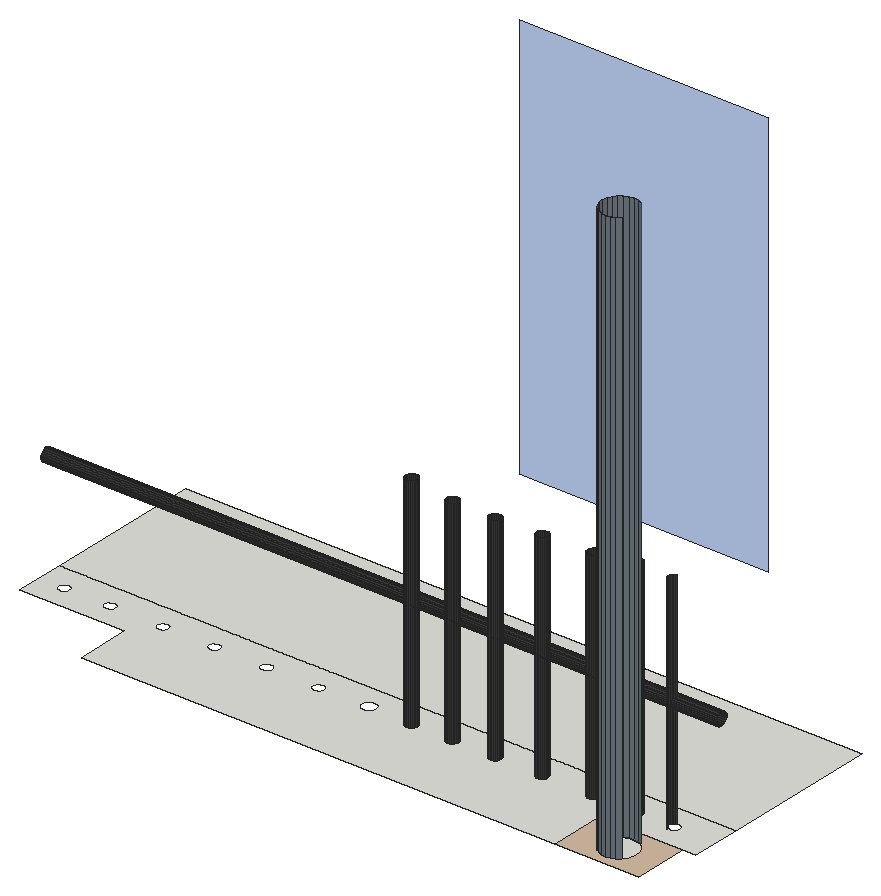
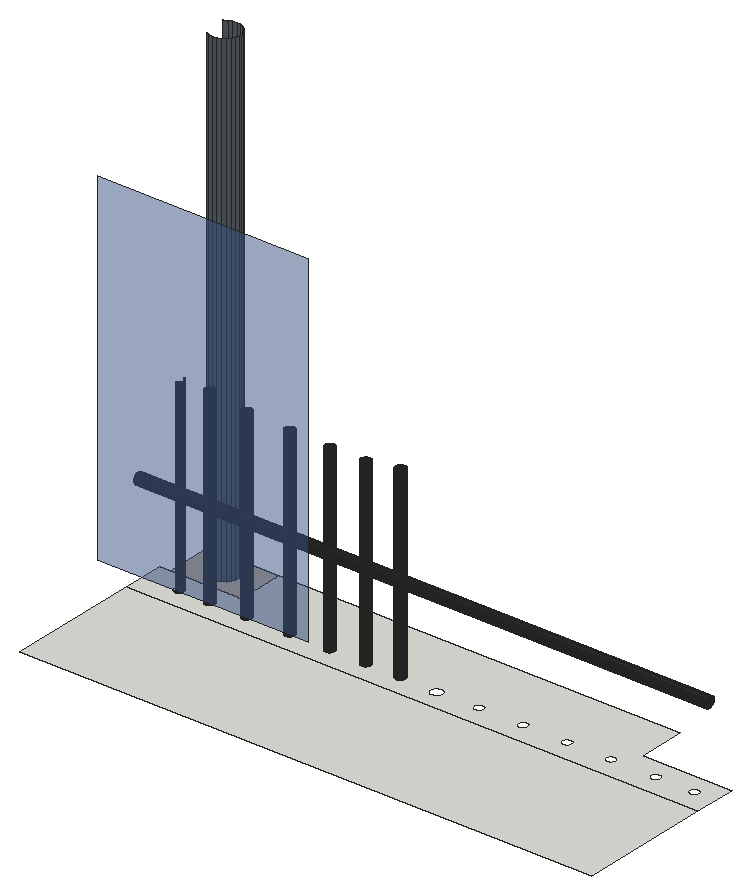
# SketchUp Ruby script. Lengths in inches.
U = 1.inch
M = Sketchup.active_model
def pt(a) = Geom::Point3d.new(a.map { |v| v * U })
def face(e, loops, mat)
  f = e.add_face(loops[0].map { |a| pt(a) })
  loops[1..].each { |l| e.add_face(l.map { |a| pt(a) }).erase! }
  f.material = f.back_material = mat if mat
  f
end
# faces: each face lists its corners as indices into pts; further lists are holes
def faces(e, pts, list, mat = nil) = list.each { |f| face(e, (f[0].is_a?(Array) ? f : [f]).map { |l| l.map { |i| pts[i] } }, mat) }
# xy, xz, yz: faces in a plane at the given z, y or x. An outline is a flat list of corners, or four numbers for a rectangle; further outlines are holes
def ring(l) = l.size == 4 ? [[l[0], l[1]], [l[2], l[1]], [l[2], l[3]], [l[0], l[3]]] : l.each_slice(2).to_a
def flat(e, list, mat, &to3) = list.each { |f| face(e, (f[0].is_a?(Array) ? f : [f]).map { |l| ring(l).map { |u, v| to3.(u, v) } }, mat) }
def xy(e, z, list, mat = nil) = flat(e, list, mat) { |x, y| [x, y, z] }
def xz(e, y, list, mat = nil) = flat(e, list, mat) { |x, z| [x, y, z] }
def yz(e, x, list, mat = nil) = flat(e, list, mat) { |y, z| [x, y, z] }
def lines(e, pts, list) = list.each { |a, b| e.add_line(pt(pts[a]), pt(pts[b])) }
# prism: a flat outline (further loops are holes) pulled along v
def prism(e, loops, v, mat = nil)
  f = face(e, loops, mat); d = Geom::Vector3d.new(v.map { |x| x * U })
  f.pushpull(f.normal.samedirection?(d) ? d.length : -d.length)
end
def box(e, o, s, mat = nil) = prism(e, [[o, [o[0] + s[0], o[1], o[2]], [o[0] + s[0], o[1] + s[1], o[2]], [o[0], o[1] + s[1], o[2]]]], [0, 0, s[2]], mat)
def at(x, y, z, deg = 0) = Geom::Transformation.translation(pt([x, y, z])) * Geom::Transformation.rotation(ORIGIN, Z_AXIS, deg.degrees)
def axes(o, x, y, z) = Geom::Transformation.new([*x, 0, *y, 0, *z, 0, *pt(o).to_a, 1])
def part(name) = M.definitions.add(name)
# library, detail: a bought-in or finely detailed component or shape, given as its bounding box
def library(name, o, s) = part(name).tap { |d| box(d.entities, o, s) }
def detail(e, o, s) = box(e.add_group.entities, o, s)
def put(e, d, t, mat = nil) = e.add_instance(d, t).tap { |i| i.material = mat if mat }
def group(e, t, mat = nil) = e.add_group.tap { |g| g.transformation = t; g.material = mat if mat }.entities
root = M.entities
M.materials.add("[Color M07]").color = [58, 58, 58]
M.materials.add("[Formica Laminate Light]").color = [213, 189, 164]
M.materials.add("[Formica Speckled Grey]").color = [112, 125, 132]
M.materials.add("[Translucent Glass Blue]").color = [85, 126, 201]
M.materials["[Translucent Glass Blue]"].alpha = 0.5
xy(root,273.71,[[[59.49,83.35,115.23,83.35,115.23,89.73,126.66,89.73,126.66,95.59,47.16,95.59,47.16,89.73,59.49,89.73],[85.8,91.86,85.57,91.89,85.36,91.97,85.18,92.11,85.04,92.29,84.95,92.5,84.92,92.73,84.95,92.96,85.04,93.17,85.18,93.35,85.36,93.49,85.57,93.58,85.8,93.61,86.02,93.58,86.24,93.49,86.42,93.35,86.56,93.17,86.64,92.96,86.67,92.73,86.64,92.5,86.56,92.29,86.42,92.11,86.24,91.97,86.02,91.89],[50.09,91.87,49.91,91.89,49.75,91.96,49.61,92.07,49.5,92.21,49.43,92.38,49.4,92.56,49.43,92.73,49.5,92.9,49.61,93.04,49.75,93.15,49.91,93.22,50.09,93.24,50.27,93.22,50.4375,93.15,50.58,93.04,50.6875,92.9,50.76,92.73,50.78,92.56,50.76,92.38,50.6875,92.21,50.58,92.07,50.4375,91.96,50.27,91.89],[55.47,91.87,55.29,91.89,55.125,91.96,54.98,92.07,54.87,92.21,54.8,92.38,54.78,92.56,54.8,92.73,54.87,92.9,54.98,93.04,55.125,93.15,55.29,93.22,55.47,93.24,55.64,93.22,55.8125,93.15,55.95,93.04,56.0625,92.9,56.13,92.73,56.15,92.56,56.13,92.38,56.0625,92.21,55.95,92.07,55.8125,91.96,55.64,91.89],[67.78,91.87,67.6,91.89,67.4375,91.96,67.29,92.07,67.18,92.21,67.12,92.38,67.09,92.56,67.12,92.73,67.18,92.9,67.29,93.04,67.4375,93.15,67.6,93.22,67.78,93.24,67.96,93.22,68.125,93.15,68.27,93.04,68.375,92.9,68.44,92.73,68.47,92.56,68.44,92.38,68.375,92.21,68.27,92.07,68.125,91.96,67.96,91.89],[61.72,91.87,61.54,91.89,61.375,91.96,61.23,92.07,61.12,92.21,61.05,92.38,61.03,92.56,61.05,92.73,61.12,92.9,61.23,93.04,61.375,93.15,61.54,93.22,61.72,93.24,61.89,93.22,62.0625,93.15,62.2,93.04,62.3125,92.9,62.38,92.73,62.4,92.56,62.38,92.38,62.3125,92.21,62.2,92.07,62.0625,91.96,61.89,91.89],[73.9,91.87,73.73,91.89,73.5625,91.96,73.42,92.07,73.31,92.21,73.24,92.38,73.22,92.56,73.24,92.73,73.31,92.9,73.42,93.04,73.5625,93.15,73.73,93.22,73.9,93.24,74.08,93.22,74.25,93.15,74.39,93.04,74.5,92.9,74.57,92.73,74.59,92.56,74.57,92.38,74.5,92.21,74.39,92.07,74.25,91.96,74.08,91.89],[121.84,91.87,121.66,91.89,121.5,91.96,121.36,92.07,121.25,92.21,121.18,92.38,121.15,92.56,121.18,92.73,121.25,92.9,121.36,93.04,121.5,93.15,121.66,93.22,121.84,93.24,122.02,93.22,122.1875,93.15,122.33,93.04,122.4375,92.9,122.51,92.73,122.53,92.56,122.51,92.38,122.4375,92.21,122.33,92.07,122.1875,91.96,122.02,91.89],[90.97,91.87,90.79,91.89,90.625,91.96,90.48,92.07,90.37,92.21,90.3,92.38,90.28,92.56,90.3,92.73,90.37,92.9,90.48,93.04,90.625,93.15,90.79,93.22,90.97,93.24,91.14,93.22,91.3125,93.15,91.45,93.04,91.5625,92.9,91.63,92.73,91.65,92.56,91.63,92.38,91.5625,92.21,91.45,92.07,91.3125,91.96,91.14,91.89],[117.47,91.87,117.29,91.89,117.125,91.96,116.98,92.07,116.87,92.21,116.8,92.38,116.78,92.56,116.8,92.73,116.87,92.9,116.98,93.04,117.125,93.15,117.29,93.22,117.47,93.24,117.64,93.22,117.8125,93.15,117.95,93.04,118.0625,92.9,118.13,92.73,118.15,92.56,118.13,92.38,118.0625,92.21,117.95,92.07,117.8125,91.96,117.64,91.89],[95.78,91.87,95.6,91.89,95.4375,91.96,95.29,92.07,95.18,92.21,95.12,92.38,95.09,92.56,95.12,92.73,95.18,92.9,95.29,93.04,95.4375,93.15,95.6,93.22,95.78,93.24,95.96,93.22,96.125,93.15,96.27,93.04,96.375,92.9,96.44,92.73,96.47,92.56,96.44,92.38,96.375,92.21,96.27,92.07,96.125,91.96,95.96,91.89],[112.34,91.87,112.16,91.89,112,91.96,111.86,92.07,111.75,92.21,111.68,92.38,111.65,92.56,111.68,92.73,111.75,92.9,111.86,93.04,112,93.15,112.16,93.22,112.34,93.24,112.52,93.22,112.6875,93.15,112.83,93.04,112.9375,92.9,113.01,92.73,113.03,92.56,113.01,92.38,112.9375,92.21,112.83,92.07,112.6875,91.96,112.52,91.89],[100.78,91.87,100.6,91.89,100.4375,91.96,100.29,92.07,100.18,92.21,100.12,92.38,100.09,92.56,100.12,92.73,100.18,92.9,100.29,93.04,100.4375,93.15,100.6,93.22,100.78,93.24,100.96,93.22,101.125,93.15,101.27,93.04,101.375,92.9,101.44,92.73,101.47,92.56,101.44,92.38,101.375,92.21,101.27,92.07,101.125,91.96,100.96,91.89],[106.34,91.87,106.16,91.89,106,91.96,105.86,92.07,105.75,92.21,105.68,92.38,105.65,92.56,105.68,92.73,105.75,92.9,105.86,93.04,106,93.15,106.16,93.22,106.34,93.24,106.52,93.22,106.6875,93.15,106.83,93.04,106.9375,92.9,107.01,92.73,107.03,92.56,107.01,92.38,106.9375,92.21,106.83,92.07,106.6875,91.96,106.52,91.89],[80.03,91.87,79.85,91.89,79.6875,91.96,79.54,92.07,79.43,92.21,79.37,92.38,79.34,92.56,79.37,92.73,79.43,92.9,79.54,93.04,79.6875,93.15,79.85,93.22,80.03,93.24,80.21,93.22,80.375,93.15,80.52,93.04,80.625,92.9,80.69,92.73,80.72,92.56,80.69,92.38,80.625,92.21,80.52,92.07,80.375,91.96,80.21,91.89]],[120.4,84.29,119.86,84.36,119.37,84.57,118.9375,84.89,118.61,85.32,118.41,85.82,118.33,86.35,118.41,86.89,118.61,87.38,118.9375,87.8125,119.37,88.14,119.86,88.35,120.4,88.42,120.93,88.35,121.43,88.14,121.86,87.8125,122.18,87.38,122.39,86.89,122.46,86.35,122.39,85.82,122.18,85.32,121.86,84.89,121.43,84.57,120.93,84.36],[90.97,91.87,90.79,91.89,90.625,91.96,90.48,92.07,90.37,92.21,90.3,92.38,90.28,92.56,90.3,92.73,90.37,92.9,90.48,93.04,90.625,93.15,90.79,93.22,90.97,93.24,91.14,93.22,91.3125,93.15,91.45,93.04,91.5625,92.9,91.63,92.73,91.65,92.56,91.63,92.38,91.5625,92.21,91.45,92.07,91.3125,91.96,91.14,91.89],[95.78,91.87,95.6,91.89,95.4375,91.96,95.29,92.07,95.18,92.21,95.12,92.38,95.09,92.56,95.12,92.73,95.18,92.9,95.29,93.04,95.4375,93.15,95.6,93.22,95.78,93.24,95.96,93.22,96.125,93.15,96.27,93.04,96.375,92.9,96.44,92.73,96.47,92.56,96.44,92.38,96.375,92.21,96.27,92.07,96.125,91.96,95.96,91.89],[100.78,91.87,100.6,91.89,100.4375,91.96,100.29,92.07,100.18,92.21,100.12,92.38,100.09,92.56,100.12,92.73,100.18,92.9,100.29,93.04,100.4375,93.15,100.6,93.22,100.78,93.24,100.96,93.22,101.125,93.15,101.27,93.04,101.375,92.9,101.44,92.73,101.47,92.56,101.44,92.38,101.375,92.21,101.27,92.07,101.125,91.96,100.96,91.89],
  [106.34,91.87,106.16,91.89,106,91.96,105.86,92.07,105.75,92.21,105.68,92.38,105.65,92.56,105.68,92.73,105.75,92.9,105.86,93.04,106,93.15,106.16,93.22,106.34,93.24,106.52,93.22,106.6875,93.15,106.83,93.04,106.9375,92.9,107.01,92.73,107.03,92.56,107.01,92.38,106.9375,92.21,106.83,92.07,106.6875,91.96,106.52,91.89],[112.34,91.87,112.16,91.89,112,91.96,111.86,92.07,111.75,92.21,111.68,92.38,111.65,92.56,111.68,92.73,111.75,92.9,111.86,93.04,112,93.15,112.16,93.22,112.34,93.24,112.52,93.22,112.6875,93.15,112.83,93.04,112.9375,92.9,113.01,92.73,113.03,92.56,113.01,92.38,112.9375,92.21,112.83,92.07,112.6875,91.96,112.52,91.89],[117.47,91.87,117.29,91.89,117.125,91.96,116.98,92.07,116.87,92.21,116.8,92.38,116.78,92.56,116.8,92.73,116.87,92.9,116.98,93.04,117.125,93.15,117.29,93.22,117.47,93.24,117.64,93.22,117.8125,93.15,117.95,93.04,118.0625,92.9,118.13,92.73,118.15,92.56,118.13,92.38,118.0625,92.21,117.95,92.07,117.8125,91.96,117.64,91.89],[47.16,95.59,126.66,114.1]])
xy(root,273.71,[[[115.23,83.35,125.11,89.73],[120.4,84.29,119.86,84.36,119.37,84.57,118.9375,84.89,118.61,85.32,118.41,85.82,118.33,86.35,118.41,86.89,118.61,87.38,118.9375,87.8125,119.37,88.14,119.86,88.35,120.4,88.42,120.93,88.35,121.43,88.14,121.86,87.8125,122.18,87.38,122.39,86.89,122.46,86.35,122.39,85.82,122.18,85.32,121.86,84.89,121.43,84.57,120.93,84.36]]],"[Formica Laminate Light]")
xz(root,114.1,[[86.49,288.95,115.77,336.88]],"[Translucent Glass Blue]")
p = [[119.86,84.36,273.71],[120.4,84.29,273.71],[120.4,84.29,341.31],[119.86,84.36,341.31],[120.93,84.36,273.71],[120.93,84.36,341.31],
  [119.37,84.57,273.71],[119.37,84.57,341.31],[121.43,84.57,273.71],[121.43,84.57,341.31],[118.9375,84.89,273.71],[118.9375,84.89,341.31],
  [121.86,84.89,273.71],[121.86,84.89,341.31],[118.61,85.32,273.71],[118.61,85.32,341.31],[118.41,85.82,273.71],[118.41,85.82,341.31],
  [118.33,86.35,273.71],[118.33,86.35,341.31],[118.41,86.89,273.71],[118.41,86.89,341.31],[118.61,87.38,273.71],[118.61,87.38,341.31],
  [118.9375,87.8125,273.71],[118.9375,87.8125,341.31],[119.37,88.14,273.71],[119.37,88.14,341.31],[119.86,88.35,273.71],[119.86,88.35,341.31],
  [121.43,88.14,273.71],[120.93,88.35,273.71],[120.93,88.35,341.31],[121.43,88.14,341.31],[120.4,88.42,273.71],[120.4,88.42,341.31],
  [90.625,91.96,273.71],[90.79,91.89,273.71],[90.79,91.89,299.74],[90.625,91.96,299.74],[90.97,91.87,273.71],[90.97,91.87,299.74],
  [91.14,91.89,273.71],[91.14,91.89,299.74],[91.3125,91.96,273.71],[91.3125,91.96,299.74],[95.4375,91.96,273.71],[95.6,91.89,273.71],
  [95.6,91.89,299.02],[95.4375,91.96,299.02],[95.78,91.87,273.71],[95.78,91.87,299.02],[95.96,91.89,273.71],[95.96,91.89,299.02],
  [96.125,91.96,273.71],[96.125,91.96,299.02],[100.4375,91.96,273.71],[100.6,91.89,273.71],[100.6,91.89,298.96],[100.4375,91.96,298.96],
  [100.78,91.87,273.71],[100.78,91.87,298.96],[100.96,91.89,273.71],[100.96,91.89,298.96],[101.125,91.96,273.71],[101.125,91.96,298.96],
  [106,91.96,273.71],[106.16,91.89,273.71],[106.16,91.89,299.14],[106,91.96,299.14],[106.34,91.87,273.71],[106.34,91.87,299.14],
  [106.52,91.89,273.71],[106.52,91.89,299.14],[106.6875,91.96,273.71],[106.6875,91.96,299.14],[112,91.96,273.71],[112.16,91.89,273.71],
  [112.16,91.89,299.39],[112,91.96,299.39],[112.34,91.87,273.71],[112.34,91.87,299.39],[112.52,91.89,273.71],[112.52,91.89,299.39],
  [112.6875,91.96,273.71],[112.6875,91.96,299.39],[117.125,91.96,273.71],[117.29,91.89,273.71],[117.29,91.89,300.16],[117.125,91.96,300.16],
  [117.47,91.87,273.71],[117.47,91.87,300.16],[117.64,91.89,273.71],[117.64,91.89,300.16],[117.8125,91.96,273.71],[117.8125,91.96,300.16],
  [121.5,91.96,273.71],[121.66,91.89,273.71],[121.66,91.89,299.96],[121.5,91.96,299.96],[90.48,92.07,273.71],[90.48,92.07,299.74],
  [91.45,92.07,273.71],[91.45,92.07,299.74],[95.29,92.07,273.71],[95.29,92.07,299.02],[96.27,92.07,273.71],[96.27,92.07,299.02],
  [100.29,92.07,273.71],[100.29,92.07,298.96],[101.27,92.07,273.71],[101.27,92.07,298.96],[105.86,92.07,273.71],[105.86,92.07,299.14],
  [106.83,92.07,273.71],[106.83,92.07,299.14],[111.86,92.07,273.71],[111.86,92.07,299.39],[112.83,92.07,273.71],[112.83,92.07,299.39],
  [116.98,92.07,273.71],[116.98,92.07,300.16],[117.95,92.07,273.71],[117.95,92.07,300.16],[121.36,92.07,273.71],[121.36,92.07,299.96],
  [90.37,92.21,273.71],[90.37,92.21,299.74],[91.5625,92.21,273.71],[91.5625,92.21,299.74],[95.18,92.21,273.71],[95.18,92.21,299.02],
  [96.375,92.21,273.71],[96.375,92.21,299.02],[100.18,92.21,273.71],[100.18,92.21,298.96],[101.375,92.21,273.71],[101.375,92.21,298.96],
  [105.75,92.21,273.71],[105.75,92.21,299.14],[106.9375,92.21,273.71],[106.9375,92.21,299.14],[111.75,92.21,273.71],[111.75,92.21,299.39],
  [112.9375,92.21,273.71],[112.9375,92.21,299.39],[116.87,92.21,273.71],[116.87,92.21,300.16],[118.0625,92.21,273.71],[118.0625,92.21,300.16],
  [121.25,92.21,273.71],[121.25,92.21,299.96],[90.3,92.38,273.71],[90.3,92.38,299.74],[91.63,92.38,273.71],[91.63,92.38,299.74],
  [95.12,92.38,273.71],[95.12,92.38,299.02],[96.44,92.38,273.71],[96.44,92.38,299.02],[100.12,92.38,273.71],[100.12,92.38,298.96],
  [101.44,92.38,273.71],[101.44,92.38,298.96],[105.68,92.38,273.71],[105.68,92.38,299.14],[107.01,92.38,273.71],[107.01,92.38,299.14],
  [111.68,92.38,273.71],[111.68,92.38,299.39],[113.01,92.38,273.71],[113.01,92.38,299.39],[116.8,92.38,273.71],[116.8,92.38,300.16],
  [118.13,92.38,273.71],[118.13,92.38,300.16],[121.18,92.38,273.71],[121.18,92.38,299.96],[90.28,92.56,273.71],[90.28,92.56,299.74],
  [91.65,92.56,273.71],[91.65,92.56,299.74],[95.09,92.56,273.71],[95.09,92.56,299.02],[96.47,92.56,273.71],[96.47,92.56,299.02],
  [100.09,92.56,273.71],[100.09,92.56,298.96],[101.47,92.56,273.71],[101.47,92.56,298.96],[105.65,92.56,273.71],[105.65,92.56,299.14],
  [107.03,92.56,273.71],[107.03,92.56,299.14],[111.65,92.56,273.71],[111.65,92.56,299.39],[113.03,92.56,273.71],[113.03,92.56,299.39],
  [116.78,92.56,273.71],[116.78,92.56,300.16],[118.15,92.56,273.71],[118.15,92.56,300.16],[121.15,92.56,273.71],[121.15,92.56,299.96],
  [90.3,92.73,273.71],[90.3,92.73,299.74],[91.63,92.73,273.71],[91.63,92.73,299.74],[95.12,92.73,273.71],[95.12,92.73,299.02],
  [96.44,92.73,273.71],[96.44,92.73,299.02],[100.12,92.73,273.71],[100.12,92.73,298.96],[101.44,92.73,273.71],[101.44,92.73,298.96],
  [105.68,92.73,273.71],[105.68,92.73,299.14],[107.01,92.73,273.71],[107.01,92.73,299.14],[111.68,92.73,273.71],[111.68,92.73,299.39],
  [113.01,92.73,273.71],[113.01,92.73,299.39],[116.8,92.73,273.71],[116.8,92.73,300.16],[118.13,92.73,273.71],[118.13,92.73,300.16],
  [121.18,92.73,273.71],[121.18,92.73,299.96],[90.37,92.9,273.71],[90.37,92.9,299.74],[91.5625,92.9,273.71],[91.5625,92.9,299.74],
  [95.18,92.9,273.71],[95.18,92.9,299.02],[96.375,92.9,273.71],[96.375,92.9,299.02],[100.18,92.9,273.71],[100.18,92.9,298.96],
  [101.375,92.9,273.71],[101.375,92.9,298.96],[105.75,92.9,273.71],[105.75,92.9,299.14],[106.9375,92.9,273.71],[106.9375,92.9,299.14],
  [111.75,92.9,273.71],[111.75,92.9,299.39],[112.9375,92.9,273.71],[112.9375,92.9,299.39],[116.87,92.9,273.71],[116.87,92.9,300.16],
  [118.0625,92.9,273.71],[118.0625,92.9,300.16],[121.25,92.9,273.71],[121.25,92.9,299.96],[90.48,93.04,273.71],[90.48,93.04,299.74],
  [91.45,93.04,273.71],[91.45,93.04,299.74],[95.29,93.04,273.71],[95.29,93.04,299.02],[96.27,93.04,273.71],[96.27,93.04,299.02],
  [100.29,93.04,273.71],[100.29,93.04,298.96],[101.27,93.04,273.71],[101.27,93.04,298.96],[105.86,93.04,273.71],[105.86,93.04,299.14],
  [106.83,93.04,273.71],[106.83,93.04,299.14],[111.86,93.04,273.71],[111.86,93.04,299.39],[112.83,93.04,273.71],[112.83,93.04,299.39],
  [116.98,93.04,273.71],[116.98,93.04,300.16],[117.95,93.04,273.71],[117.95,93.04,300.16],[121.36,93.04,273.71],[121.36,93.04,299.96],
  [90.625,93.15,273.71],[90.625,93.15,299.74],[91.3125,93.15,273.71],[91.3125,93.15,299.74],[95.4375,93.15,273.71],[95.4375,93.15,299.02],
  [96.125,93.15,273.71],[96.125,93.15,299.02],[100.4375,93.15,273.71],[100.4375,93.15,298.96],[101.125,93.15,273.71],[101.125,93.15,298.96],
  [106,93.15,273.71],[106,93.15,299.14],[106.6875,93.15,273.71],[106.6875,93.15,299.14],[112,93.15,273.71],[112,93.15,299.39],
  [112.6875,93.15,273.71],[112.6875,93.15,299.39],[117.125,93.15,273.71],[117.125,93.15,300.16],[117.8125,93.15,273.71],[117.8125,93.15,300.16],
  [121.5,93.15,273.71],[121.5,93.15,299.96],[90.79,93.22,273.71],[90.79,93.22,299.74],[90.97,93.24,273.71],[90.97,93.24,299.74],
  [91.14,93.22,273.71],[91.14,93.22,299.74],[95.6,93.22,273.71],[95.6,93.22,299.02],[95.78,93.24,273.71],[95.78,93.24,299.02],
  [95.96,93.22,273.71],[95.96,93.22,299.02],[100.6,93.22,273.71],[100.6,93.22,298.96],[100.78,93.24,273.71],[100.78,93.24,298.96],
  [100.96,93.22,273.71],[100.96,93.22,298.96],[106.16,93.22,273.71],[106.16,93.22,299.14],[106.34,93.24,273.71],[106.34,93.24,299.14],
  [106.52,93.22,273.71],[106.52,93.22,299.14],[112.16,93.22,273.71],[112.16,93.22,299.39],[112.34,93.24,273.71],[112.34,93.24,299.39],
  [112.52,93.22,273.71],[112.52,93.22,299.39],[117.29,93.22,273.71],[117.29,93.22,300.16],[117.47,93.24,273.71],[117.47,93.24,300.16],
  [117.64,93.22,273.71],[117.64,93.22,300.16],[121.66,93.22,273.71],[121.66,93.22,299.96],[126.66,93.33,285.64],[126.66,93.15,285.72],
  [47.16,93.15,285.72],[47.16,93.33,285.64],[126.66,93.52,285.62],[47.16,93.52,285.62],[126.66,93.72,285.64],[47.16,93.72,285.64],
  [126.66,93.9,285.72],[47.16,93.9,285.72],[126.66,92.99,285.84],[47.16,92.99,285.84],[126.66,94.05,285.84],[47.16,94.05,285.84],
  [126.66,92.875,285.99],[47.16,92.875,285.99],[126.66,94.17,285.99],[47.16,94.17,285.99],[126.66,92.8,286.17],[47.16,92.8,286.17],
  [126.66,94.25,286.17],[47.16,94.25,286.17],[126.66,92.77,286.37],[47.16,92.77,286.37],[126.66,94.27,286.37],[47.16,94.27,286.37],
  [126.66,92.8,286.5625],[47.16,92.8,286.5625],[126.66,94.25,286.5625],[47.16,94.25,286.5625],[126.66,92.875,286.74],[47.16,92.875,286.74],
  [126.66,94.17,286.74],[47.16,94.17,286.74],[126.66,92.99,286.9],[47.16,92.99,286.9],[126.66,94.05,286.9],[47.16,94.05,286.9],
  [126.66,93.15,287.02],[47.16,93.15,287.02],[126.66,93.9,287.02],[47.16,93.9,287.02],[126.66,93.33,287.09],[47.16,93.33,287.09],
  [126.66,93.72,287.09],[47.16,93.72,287.09],[126.66,93.52,287.12],[47.16,93.52,287.12]]
faces(root,p,[[0,1,2,3],[1,4,5,2],[6,0,3,7],[4,8,9,5],[10,6,7,11],[8,12,13,9],[14,10,11,15],[16,14,15,17],
  [18,16,17,19],[20,18,19,21],[22,20,21,23],[24,22,23,25],[26,24,25,27],[28,26,27,29],[30,31,32,33],[34,28,29,35],
  [31,34,35,32]],"[Formica Speckled Grey]")
faces(root,p,[[36,37,38,39],[37,40,41,38],[40,42,43,41],[42,44,45,43],[46,47,48,49],[47,50,51,48],[50,52,53,51],[52,54,55,53],
  [56,57,58,59],[57,60,61,58],[60,62,63,61],[62,64,65,63],[66,67,68,69],[67,70,71,68],[70,72,73,71],[72,74,75,73],
  [76,77,78,79],[77,80,81,78],[80,82,83,81],[82,84,85,83],[86,87,88,89],[87,90,91,88],[90,92,93,91],[92,94,95,93],
  [96,97,98,99],[100,36,39,101],[44,102,103,45],[104,46,49,105],[54,106,107,55],[108,56,59,109],[64,110,111,65],[112,66,69,113],
  [74,114,115,75],[116,76,79,117],[84,118,119,85],[120,86,89,121],[94,122,123,95],[124,96,99,125],[126,100,101,127],[102,128,129,103],
  [130,104,105,131],[106,132,133,107],[134,108,109,135],[110,136,137,111],[138,112,113,139],[114,140,141,115],[142,116,117,143],[118,144,145,119],
  [146,120,121,147],[122,148,149,123],[150,124,125,151],[152,126,127,153],[128,154,155,129],[156,130,131,157],[132,158,159,133],[160,134,135,161],
  [136,162,163,137],[164,138,139,165],[140,166,167,141],[168,142,143,169],[144,170,171,145],[172,146,147,173],[148,174,175,149],[176,150,151,177],
  [178,152,153,179],[154,180,181,155],[182,156,157,183],[158,184,185,159],[186,160,161,187],[162,188,189,163],[190,164,165,191],[166,192,193,167],
  [194,168,169,195],[170,196,197,171],[198,172,173,199],[174,200,201,175],[202,176,177,203],[204,178,179,205],[180,206,207,181],[208,182,183,209],
  [184,210,211,185],[212,186,187,213],[188,214,215,189],[216,190,191,217],[192,218,219,193],[220,194,195,221],[196,222,223,197],[224,198,199,225],
  [200,226,227,201],[228,202,203,229],[230,204,205,231],[206,232,233,207],[234,208,209,235],[210,236,237,211],[238,212,213,239],[214,240,241,215],
  [242,216,217,243],[218,244,245,219],[246,220,221,247],[222,248,249,223],[250,224,225,251],[226,252,253,227],[254,228,229,255],[256,230,231,257],
  [232,258,259,233],[260,234,235,261],[236,262,263,237],[264,238,239,265],[240,266,267,241],[268,242,243,269],[244,270,271,245],[272,246,247,273],
  [248,274,275,249],[276,250,251,277],[252,278,279,253],[280,254,255,281],[282,256,257,283],[258,284,285,259],[286,260,261,287],[262,288,289,263],
  [290,264,265,291],[266,292,293,267],[294,268,269,295],[270,296,297,271],[298,272,273,299],[274,300,301,275],[302,276,277,303],[278,304,305,279],
  [306,280,281,307],[308,282,283,309],[310,308,309,311],[312,310,311,313],[284,312,313,285],[314,286,287,315],[316,314,315,317],[318,316,317,319],
  [288,318,319,289],[320,290,291,321],[322,320,321,323],[324,322,323,325],[292,324,325,293],[326,294,295,327],[328,326,327,329],[330,328,329,331],
  [296,330,331,297],[332,298,299,333],[334,332,333,335],[336,334,335,337],[300,336,337,301],[338,302,303,339],[340,338,339,341],[342,340,341,343],
  [304,342,343,305],[344,306,307,345],[346,347,348,349],[350,346,349,351],[352,350,351,353],[354,352,353,355],[347,356,357,348],[358,354,355,359],
  [356,360,361,357],[362,358,359,363],[360,364,365,361],[366,362,363,367],[364,368,369,365],[370,366,367,371],[368,372,373,369],[374,370,371,375],
  [372,376,377,373],[378,374,375,379],[376,380,381,377],[382,378,379,383],[380,384,385,381],[386,382,383,387],[384,388,389,385],[390,386,387,391],
  [388,392,393,389],[392,390,391,393]],"[Color M07]")
